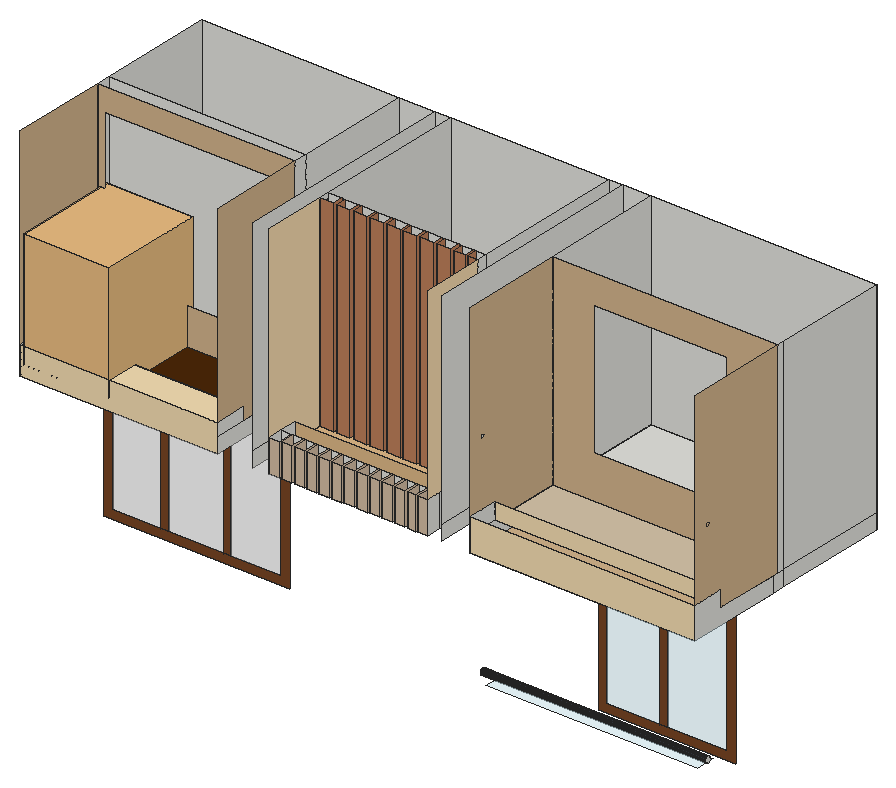
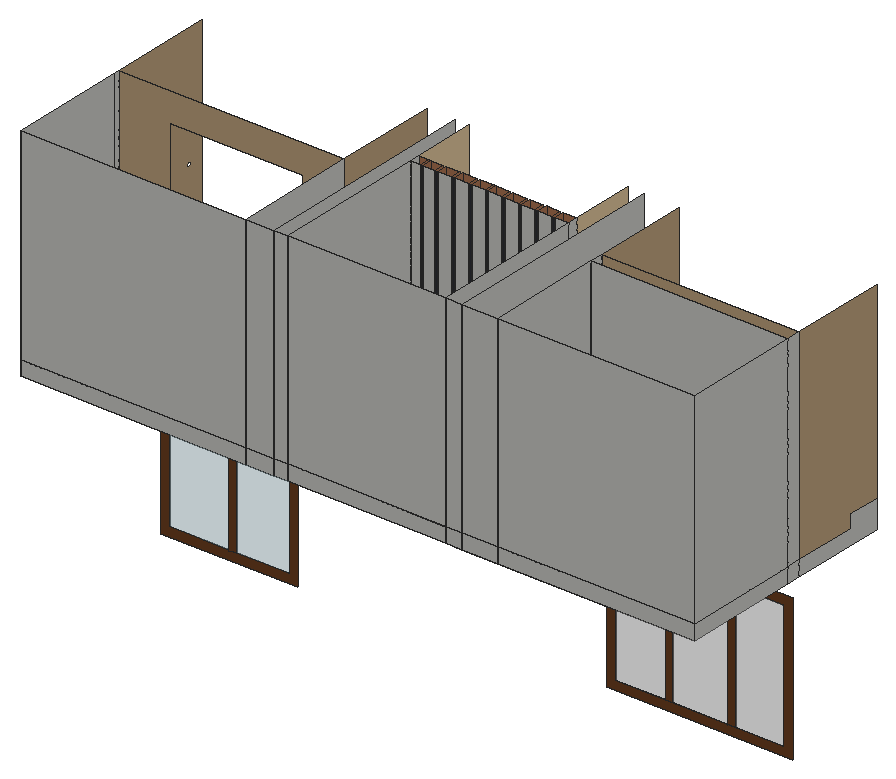
# SketchUp Ruby script. Lengths in inches.
U = 1.inch
M = Sketchup.active_model
def pt(a) = Geom::Point3d.new(a.map { |v| v * U })
def face(e, loops, mat)
  f = e.add_face(loops[0].map { |a| pt(a) })
  loops[1..].each { |l| e.add_face(l.map { |a| pt(a) }).erase! }
  f.material = f.back_material = mat if mat
  f
end
# faces: each face lists its corners as indices into pts; further lists are holes
def faces(e, pts, list, mat = nil) = list.each { |f| face(e, (f[0].is_a?(Array) ? f : [f]).map { |l| l.map { |i| pts[i] } }, mat) }
# xy, xz, yz: faces in a plane at the given z, y or x. An outline is a flat list of corners, or four numbers for a rectangle; further outlines are holes
def ring(l) = l.size == 4 ? [[l[0], l[1]], [l[2], l[1]], [l[2], l[3]], [l[0], l[3]]] : l.each_slice(2).to_a
def flat(e, list, mat, &to3) = list.each { |f| face(e, (f[0].is_a?(Array) ? f : [f]).map { |l| ring(l).map { |u, v| to3.(u, v) } }, mat) }
def xy(e, z, list, mat = nil) = flat(e, list, mat) { |x, y| [x, y, z] }
def xz(e, y, list, mat = nil) = flat(e, list, mat) { |x, z| [x, y, z] }
def yz(e, x, list, mat = nil) = flat(e, list, mat) { |y, z| [x, y, z] }
def lines(e, pts, list) = list.each { |a, b| e.add_line(pt(pts[a]), pt(pts[b])) }
# prism: a flat outline (further loops are holes) pulled along v
def prism(e, loops, v, mat = nil)
  f = face(e, loops, mat); d = Geom::Vector3d.new(v.map { |x| x * U })
  f.pushpull(f.normal.samedirection?(d) ? d.length : -d.length)
end
def box(e, o, s, mat = nil) = prism(e, [[o, [o[0] + s[0], o[1], o[2]], [o[0] + s[0], o[1] + s[1], o[2]], [o[0], o[1] + s[1], o[2]]]], [0, 0, s[2]], mat)
def at(x, y, z, deg = 0) = Geom::Transformation.translation(pt([x, y, z])) * Geom::Transformation.rotation(ORIGIN, Z_AXIS, deg.degrees)
def axes(o, x, y, z) = Geom::Transformation.new([*x, 0, *y, 0, *z, 0, *pt(o).to_a, 1])
def part(name) = M.definitions.add(name)
# library, detail: a bought-in or finely detailed component or shape, given as its bounding box
def library(name, o, s) = part(name).tap { |d| box(d.entities, o, s) }
def detail(e, o, s) = box(e.add_group.entities, o, s)
def put(e, d, t, mat = nil) = e.add_instance(d, t).tap { |i| i.material = mat if mat }
def group(e, t, mat = nil) = e.add_group.tap { |g| g.transformation = t; g.material = mat if mat }.entities
root = M.entities
M.materials.add("[0027_PeachPuff]").color = [255, 218, 185]
M.materials.add("[0034_Wheat]").color = [245, 222, 179]
M.materials.add("[0035_Tan]").color = [210, 180, 140]
M.materials.add("[0036_BurlyWood]1").color = [222, 184, 135]
M.materials.add("[Formica Beige]").color = [247, 219, 174]
M.materials.add("[Formica Laminate Dark]").color = [50, 53, 60]
M.materials.add("[Formica Laminate Light]").color = [213, 189, 164]
M.materials.add("[Leather Red Brown]").color = [76, 40, 8]
M.materials.add("[Tile Various Tan]").color = [214, 196, 169]
M.materials.add("[Translucent Glass Gray]").color = [191, 191, 191]
M.materials["[Translucent Glass Gray]"].alpha = 0.5
M.materials.add("[Translucent Glass Safety]").color = [204, 235, 244]
M.materials["[Translucent Glass Safety]"].alpha = 0.5
M.materials.add("[Wood Veneer 01]").color = [120, 70, 37]
M.materials.add("[Wood Veneer 02]").color = [190, 128, 91]
c1 = library("chau cay",[-24.34,-109.24,0],[56.46,62.58,79.69])
xy(root,3433.875,[[1418.67,332.12,2047.84,393.82]],"[Translucent Glass Safety]")
xy(root,3459.4375,[[2057.02,340.46,2059.25,340.76,2061.33,341.62,2063.12,342.99,2064.49,344.77,2065.35,346.85,2065.64,349.09,2065.35,351.32,2064.6,353.14,2049.4375,353.14,2048.6875,351.32,2048.39,349.09,2048.6875,346.85,2049.55,344.77,2050.92,342.99,2052.7,341.62,2054.79,340.76],[2049.4375,353.14,2064.6,353.14,2064.49,353.4,2063.12,355.1875,2061.33,356.56,2059.25,357.42,2057.02,357.71,2054.79,357.42,2052.7,356.56,2050.92,355.1875,2049.55,353.4]])
xy(root,3461.67,[[1409.52,340.46,1411.75,340.76,1413.83,341.62,1415.62,342.99,1416.99,344.77,1417.85,346.85,1418.14,349.09,1417.85,351.32,1417.22,352.84,1401.82,352.84,1401.1875,351.32,1400.89,349.09,1401.1875,346.85,1402.05,344.77,1403.42,342.99,1405.2,341.62,1407.29,340.76],[1401.82,352.84,1417.22,352.84,1416.99,353.4,1415.62,355.1875,1413.83,356.56,1411.75,357.42,1409.52,357.71,1407.29,357.42,1405.2,356.56,1403.42,355.1875,1402.05,353.4]])
xy(root,3798.8125,[[800.41,509.42,800.41,584.29,1272.8,584.29,1272.8,548.04,1258.16,548.04,1258.16,509.42,1201.66,509.42,1201.66,548.04,1191.29,548.04,1191.29,509.42,1134.78,509.42,1134.78,548.04,1124.41,548.04,1124.41,509.42,1067.91,509.42,1067.91,548.04,1057.54,548.04,1057.54,509.42,1001.03,509.42,1001.03,548.04,990.66,548.04,990.66,509.42,934.16,509.42,934.16,548.04,923.79,548.04,923.79,509.42,867.28,509.42,867.28,548.04,856.91,548.04,856.91,509.42],[800.41,509.42,856.91,548.04],[867.28,509.42,923.79,548.04],[934.16,509.42,990.66,548.04],[1001.03,509.42,1057.54,548.04],
  [1067.91,509.42,1124.41,548.04],[1134.78,509.42,1191.29,548.04],[1201.66,509.42,1258.16,548.04],[800.41,548.04,1272.8,584.29],[58.44,584.29,646.67,623.89],
  [646.67,584.29,752.97,623.89],[752.97,584.29,800.41,623.89],[800.41,584.29,1272.8,623.89],[1272.8,584.29,1313.62,623.89],[1272.8,584.29,1313.62,623.89],
  [1313.62,584.29,1398.32,623.89],[58.44,623.89,646.67,971.67],[646.67,623.89,752.97,971.67],[752.97,623.89,800.41,971.67],[800.41,623.89,1272.8,971.67],
  [1272.8,623.89,1313.62,971.67],[1313.62,623.89,1398.32,971.67],[1398.32,623.89,2069.85,971.67]])
xy(root,3798.8125,[[800.41,338.63,800.41,509.42,856.91,509.42,856.91,548.04,867.28,548.04,867.28,509.42,923.79,509.42,923.79,548.04,934.16,548.04,934.16,509.42,990.66,509.42,990.66,548.04,1001.03,548.04,1001.03,509.42,1057.54,509.42,1057.54,548.04,1067.91,548.04,1067.91,509.42,1124.41,509.42,1124.41,548.04,1134.78,548.04,1134.78,509.42,1191.29,509.42,1191.29,548.04,1201.66,548.04,1201.66,509.42,1258.16,509.42,1258.16,548.04,1272.8,548.04,1272.8,338.63]],"[0027_PeachPuff]")
xy(root,3798.8125,[[58.44,295.82,646.67,584.29],[1398.32,295.82,2069.85,584.29],[1398.32,584.29,2069.85,623.89]],"[0035_Tan]")
xy(root,3798.8125,[[800.41,295.82,831.22,338.63],[837.47,295.82,868.28,338.63],[875.6,295.82,906.41,338.63],[912.41,295.82,943.22,338.63],[949.16,295.82,979.97,338.63],
  [986.78,295.82,1017.6,338.63],[1024.35,295.82,1055.16,338.63],[1062.53,295.82,1093.35,338.63],[1100.28,295.82,1131.1,338.63],[1137.66,295.82,1168.47,338.63],
  [1175.22,295.82,1206.03,338.63],[1212.97,295.82,1238.19,338.63],[1243.78,295.82,1272.8,338.63]],"[Formica Laminate Light]")
xy(root,3844,[[800.41,483.92,841.6875,514.17],[850.41,483.92,891.6875,514.17],[900.97,483.92,942.25,514.17],[949.72,483.92,991,514.17],[1000.6,483.92,1041.875,514.17],
  [1049.35,483.92,1090.625,514.17],[1099.6,483.92,1140.875,514.17],[1149.66,483.92,1190.9375,514.17],[1200.46,483.92,1235.22,514.17],[1241.74,483.92,1272.8,514.17],
  [800.41,514.17,1272.8,971.67],[58.44,584.29,646.67,623.89],[1398.32,604.09,2069.85,971.67],[58.44,623.89,646.67,971.67]])
xy(root,3844,[[800.41,390.27,1272.8,390.27,1272.8,483.92,1241.74,483.92,1241.74,514.17,1235.22,514.17,1235.22,483.92,1200.46,483.92,1200.46,514.17,1190.9375,514.17,1190.9375,483.92,1149.66,483.92,1149.66,514.17,1140.875,514.17,1140.875,483.92,1099.6,483.92,1099.6,514.17,1090.625,514.17,1090.625,483.92,1049.35,483.92,1049.35,514.17,1041.875,514.17,1041.875,483.92,1000.6,483.92,1000.6,514.17,991,514.17,991,483.92,949.72,483.92,949.72,514.17,942.25,514.17,942.25,483.92,900.97,483.92,900.97,514.17,891.6875,514.17,891.6875,483.92,850.41,483.92,850.41,514.17,841.6875,514.17,841.6875,483.92,800.41,483.92]],"[0036_BurlyWood]1")
xy(root,3844,[[58.44,390.27,646.67,584.29]],"[Leather Red Brown]")
xy(root,3844,[[1398.32,390.27,2069.85,604.09]],"[Tile Various Tan]")
xy(root,3881.75,[[58.44,295.82,646.67,390.27]],"[0034_Wheat]")
xz(root,295.82,[[58.44,3798.8125,646.67,3881.75],[1398.32,3798.8125,2069.85,3893.0625]],"[0034_Wheat]")
xz(root,295.82,[[800.41,3798.8125,831.22,3896.1875],[837.47,3798.8125,868.28,3896.1875],[875.6,3798.8125,906.41,3896.1875],[912.41,3798.8125,943.22,3896.1875],[949.16,3798.8125,979.97,3896.1875],
  [986.78,3798.8125,1017.6,3896.1875],[1024.35,3798.8125,1055.16,3896.1875],[1062.53,3798.8125,1093.35,3896.1875],[1100.28,3798.8125,1131.1,3896.1875],[1137.66,3798.8125,1168.47,3896.1875],
  [1175.22,3798.8125,1206.03,3896.1875],[1212.97,3798.8125,1238.19,3896.1875],[1243.78,3798.8125,1272.8,3896.1875]],"[Formica Laminate Light]")
xz(root,338.63,[[800.41,3798.8125,831.22,3896.1875],[837.47,3798.8125,868.28,3896.1875],[875.6,3798.8125,906.41,3896.1875],[912.41,3798.8125,943.22,3896.1875],[949.16,3798.8125,979.97,3896.1875],
  [986.78,3798.8125,1017.6,3896.1875],[1024.35,3798.8125,1055.16,3896.1875],[1062.53,3798.8125,1093.35,3896.1875],[1100.28,3798.8125,1131.1,3896.1875],[1137.66,3798.8125,1168.47,3896.1875],
  [1175.22,3798.8125,1206.03,3896.1875],[1212.97,3798.8125,1238.19,3896.1875],[1243.78,3798.8125,1272.8,3896.1875]])
xz(root,338.63,[[831.22,3798.8125,837.47,3896.1875],[868.28,3798.8125,875.6,3896.1875],[906.41,3798.8125,912.41,3896.1875],[943.22,3798.8125,949.16,3896.1875],[979.97,3798.8125,986.78,3896.1875],
  [1017.6,3798.8125,1024.35,3896.1875],[1055.16,3798.8125,1062.53,3896.1875],[1093.35,3798.8125,1100.28,3896.1875],[1131.1,3798.8125,1137.66,3896.1875],[1168.47,3798.8125,1175.22,3896.1875],
  [1206.03,3798.8125,1212.97,3896.1875],[1238.19,3798.8125,1243.78,3896.1875]],"[Formica Laminate Dark]")
xz(root,390.27,[[58.44,3844,646.67,3881.75]])
xz(root,390.27,[[1398.32,3844,2069.85,3893.0625]],"[0034_Wheat]")
xz(root,390.27,[[800.41,3844,1272.8,3896.1875]],"[0036_BurlyWood]1")
xz(root,483.92,[[800.41,3844,841.6875,4453.25],[850.41,3844,891.6875,4453.25],[900.97,3844,942.25,4453.25],[949.72,3844,991,4453.25],[1000.6,3844,1041.875,4453.25],
  [1049.35,3844,1090.625,4453.25],[1099.6,3844,1140.875,4453.25],[1149.66,3844,1190.9375,4453.25],[1200.46,3844,1235.22,4453.25],[1241.74,3844,1272.8,4453.25]],"[Wood Veneer 02]")
xz(root,514.17,[[800.41,3844,841.6875,4453.25],[850.41,3844,891.6875,4453.25],[900.97,3844,942.25,4453.25],[949.72,3844,991,4453.25],[1000.6,3844,1041.875,4453.25],
  [1049.35,3844,1090.625,4453.25],[1099.6,3844,1140.875,4453.25],[1149.66,3844,1190.9375,4453.25],[1200.46,3844,1235.22,4453.25],[1241.74,3844,1272.8,4453.25]])
xz(root,514.17,[[841.6875,3844,850.41,4453.25],[891.6875,3844,900.97,4453.25],[942.25,3844,949.72,4453.25],[991,3844,1000.6,4453.25],[1041.875,3844,1049.35,4453.25],
  [1090.625,3844,1099.6,4453.25],[1140.875,3844,1149.66,4453.25],[1190.9375,3844,1200.46,4453.25],[1235.22,3844,1241.74,4453.25]],"[Formica Laminate Dark]")
xz(root,584.29,[[[58.44,3844,646.67,4453.25],[80.45,3953.99,630.58,4386.93]]],"[0035_Tan]")
xz(root,584.29,[[102.12,3330.58,247.0625,3710.59],[269.68,3330.58,433.0625,3710.59],[455.68,3330.58,604.93,3710.59]],"[Translucent Glass Gray]")
xz(root,584.29,[[[76.9,3305.37,630.15,3735.8],[102.12,3330.58,604.93,3710.59]],[247.0625,3330.58,269.68,3710.59],[433.0625,3330.58,455.68,3710.59]],"[Wood Veneer 01]")
xz(root,604.09,[[[1398.32,3844,2069.85,4453.25],[1523.05,3973.96,1917.8,4368.71]]],"[0035_Tan]")
xz(root,623.89,[[58.44,3844,646.67,4453.25]])
xz(root,623.89,[[1546.07,3301.52,1703.52,3696.56],[1725.625,3301.52,1903.36,3696.56]],"[Translucent Glass Safety]")
xz(root,623.89,[[[1520.9,3276.35,1928.53,3721.73],[1546.07,3301.52,1903.36,3696.56]],[1703.52,3301.52,1725.625,3696.56]],"[Wood Veneer 01]")
xz(root,971.67,[[58.44,3798.8125,646.67,3844],[646.67,3798.8125,752.97,3844],[752.97,3798.8125,800.41,3844],[800.41,3798.8125,1272.8,3844],[1272.8,3798.8125,1313.62,3844],
  [1313.62,3798.8125,1398.32,3844],[1398.32,3798.8125,2069.85,3844],[58.44,3844,646.67,4453.25],[646.67,3844,752.97,4453.25],[752.97,3844,800.41,4453.25],
  [800.41,3844,1272.8,4453.25],[1272.8,3844,1313.62,4453.25],[1313.62,3844,1398.32,4453.25],[1398.32,3844,2069.85,4453.25]])
yz(root,58.44,[[295.82,3798.8125,295.82,3881.75,390.27,3881.75,390.27,3844,584.29,3844,584.29,3798.8125],[584.29,3798.8125,623.89,3844],[623.89,3798.8125,971.67,3844],[584.29,3844,623.89,4453.25],[623.89,3844,971.67,4453.25]])
yz(root,58.44,[[390.27,3844,584.29,3844,584.29,4453.25,295.82,4453.25,295.82,3881.75,390.27,3881.75]],"[0035_Tan]")
yz(root,646.67,[[295.82,3798.8125,971.67,3844],[295.82,3844,390.27,3881.75],[584.29,3844,623.89,4453.25],[623.89,3844,971.67,4453.25]])
yz(root,646.67,[[390.27,3844,390.27,3881.75,295.82,3881.75,295.82,4453.25,584.29,4453.25,584.29,3844]],"[0035_Tan]")
yz(root,752.97,[[295.82,3798.8125,971.67,3844],[295.82,3844,971.67,4453.25]])
yz(root,800.41,[[295.82,3798.8125,338.63,3896.1875],[338.63,3798.8125,971.67,3798.8125,971.67,3844,390.27,3844,390.27,3896.1875,338.63,3896.1875],[483.92,3844,514.17,4453.25],[514.17,3844,971.67,4453.25]])
yz(root,800.41,[[390.27,3844,483.92,3844,483.92,4453.25,295.82,4453.25,295.82,3896.1875,390.27,3896.1875]],"[Formica Beige]")
yz(root,831.22,[[295.82,3798.8125,338.63,3896.1875]],"[Formica Laminate Light]")
yz(root,837.47,[[295.82,3798.8125,338.63,3896.1875]],"[Formica Laminate Light]")
yz(root,841.6875,[[483.92,3844,514.17,4453.25]],"[Wood Veneer 02]")
yz(root,850.41,[[483.92,3844,514.17,4453.25]],"[Wood Veneer 02]")
yz(root,868.28,[[295.82,3798.8125,338.63,3896.1875]],"[Formica Laminate Light]")
yz(root,875.6,[[295.82,3798.8125,338.63,3896.1875]],"[Formica Laminate Light]")
yz(root,891.6875,[[483.92,3844,514.17,4453.25]],"[Wood Veneer 02]")
yz(root,900.97,[[483.92,3844,514.17,4453.25]],"[Wood Veneer 02]")
yz(root,906.41,[[295.82,3798.8125,338.63,3896.1875]],"[Formica Laminate Light]")
yz(root,912.41,[[295.82,3798.8125,338.63,3896.1875]],"[Formica Laminate Light]")
yz(root,942.25,[[483.92,3844,514.17,4453.25]],"[Wood Veneer 02]")
yz(root,943.22,[[295.82,3798.8125,338.63,3896.1875]],"[Formica Laminate Light]")
yz(root,949.16,[[295.82,3798.8125,338.63,3896.1875]],"[Formica Laminate Light]")
yz(root,949.72,[[483.92,3844,514.17,4453.25]],"[Wood Veneer 02]")
yz(root,979.97,[[295.82,3798.8125,338.63,3896.1875]],"[Formica Laminate Light]")
yz(root,986.78,[[295.82,3798.8125,338.63,3896.1875]],"[Formica Laminate Light]")
yz(root,991,[[483.92,3844,514.17,4453.25]],"[Wood Veneer 02]")
yz(root,1000.6,[[483.92,3844,514.17,4453.25]],"[Wood Veneer 02]")
yz(root,1017.6,[[295.82,3798.8125,338.63,3896.1875]],"[Formica Laminate Light]")
yz(root,1024.35,[[295.82,3798.8125,338.63,3896.1875]],"[Formica Laminate Light]")
yz(root,1041.875,[[483.92,3844,514.17,4453.25]],"[Wood Veneer 02]")
yz(root,1049.35,[[483.92,3844,514.17,4453.25]],"[Wood Veneer 02]")
yz(root,1055.16,[[295.82,3798.8125,338.63,3896.1875]],"[Formica Laminate Light]")
yz(root,1062.53,[[295.82,3798.8125,338.63,3896.1875]],"[Formica Laminate Light]")
yz(root,1090.625,[[483.92,3844,514.17,4453.25]],"[Wood Veneer 02]")
yz(root,1093.35,[[295.82,3798.8125,338.63,3896.1875]],"[Formica Laminate Light]")
yz(root,1099.6,[[483.92,3844,514.17,4453.25]],"[Wood Veneer 02]")
yz(root,1100.28,[[295.82,3798.8125,338.63,3896.1875]],"[Formica Laminate Light]")
yz(root,1131.1,[[295.82,3798.8125,338.63,3896.1875]],"[Formica Laminate Light]")
yz(root,1137.66,[[295.82,3798.8125,338.63,3896.1875]],"[Formica Laminate Light]")
yz(root,1140.875,[[483.92,3844,514.17,4453.25]],"[Wood Veneer 02]")
yz(root,1149.66,[[483.92,3844,514.17,4453.25]],"[Wood Veneer 02]")
yz(root,1168.47,[[295.82,3798.8125,338.63,3896.1875]],"[Formica Laminate Light]")
yz(root,1175.22,[[295.82,3798.8125,338.63,3896.1875]],"[Formica Laminate Light]")
yz(root,1190.9375,[[483.92,3844,514.17,4453.25]],"[Wood Veneer 02]")
yz(root,1200.46,[[483.92,3844,514.17,4453.25]],"[Wood Veneer 02]")
yz(root,1206.03,[[295.82,3798.8125,338.63,3896.1875]],"[Formica Laminate Light]")
yz(root,1212.97,[[295.82,3798.8125,338.63,3896.1875]],"[Formica Laminate Light]")
yz(root,1235.22,[[483.92,3844,514.17,4453.25]],"[Wood Veneer 02]")
yz(root,1238.19,[[295.82,3798.8125,338.63,3896.1875]],"[Formica Laminate Light]")
yz(root,1241.74,[[483.92,3844,514.17,4453.25]],"[Wood Veneer 02]")
yz(root,1243.78,[[295.82,3798.8125,338.63,3896.1875]],"[Formica Laminate Light]")
yz(root,1272.8,[[295.82,3798.8125,338.63,3896.1875],[338.63,3798.8125,338.63,3896.1875,390.27,3896.1875,390.27,3844,971.67,3844,971.67,3798.8125],[483.92,3844,514.17,4453.25],[514.17,3844,971.67,4453.25]])
yz(root,1272.8,[[390.27,3844,390.27,3896.1875,295.82,3896.1875,295.82,4453.25,483.92,4453.25,483.92,3844]],"[Formica Beige]")
yz(root,1313.62,[[295.82,3798.8125,971.67,3844],[295.82,3844,971.67,4453.25]])
yz(root,1398.32,[[295.82,3798.8125,971.67,3844],[295.82,3844,390.27,3893.0625],[604.09,3844,971.67,4453.25]])
yz(root,1398.32,[[[390.27,3844,604.09,3844,604.09,4453.25,295.82,4453.25,295.82,3893.0625,390.27,3893.0625],[343.39,4082.13,341.61,4082.37,339.95,4083.05,338.53,4084.15,337.4375,4085.57,336.75,4087.23,336.52,4089.01,336.75,4090.79,337.4375,4092.45,338.53,4093.87,339.95,4094.96,341.61,4095.65,343.39,4095.88,345.17,4095.65,346.83,4094.96,348.25,4093.87,349.34,4092.45,350.03,4090.79,350.27,4089.01,350.03,4087.23,349.34,4085.57,348.25,4084.15,346.83,4083.05,345.17,4082.37]]],"[0035_Tan]")
yz(root,2069.85,[[344.51,3450.8125,346.74,3451.11,348.82,3451.97,350.61,3453.34,351.98,3455.125,352.84,3457.21,353.14,3459.4375,352.84,3461.67,351.98,3463.75,350.61,3465.54,348.82,3466.91,346.74,3467.77,344.51,3468.0625,342.28,3467.77,340.2,3466.91,338.41,3465.54,337.04,3463.75,336.18,3461.67,335.89,3459.4375,336.18,3457.21,337.04,3455.125,338.41,3453.34,340.2,3451.97,342.28,3451.11],[295.82,3798.8125,584.29,3798.8125,584.29,3844,390.27,3844,390.27,3893.0625,295.82,3893.0625],[584.29,3798.8125,623.89,3844],[623.89,3798.8125,971.67,3844],[604.09,3844,623.89,4453.25],
  [623.89,3844,971.67,4453.25]])
yz(root,2069.85,[[[390.27,3844,390.27,3893.0625,295.82,3893.0625,295.82,4453.25,604.09,4453.25,604.09,3844],[343.39,4082.13,345.17,4082.37,346.83,4083.05,348.25,4084.15,349.34,4085.57,350.03,4087.23,350.27,4089.01,350.03,4090.79,349.34,4092.45,348.25,4093.87,346.83,4094.96,345.17,4095.65,343.39,4095.88,341.61,4095.65,339.95,4094.96,338.53,4093.87,337.4375,4092.45,336.75,4090.79,336.52,4089.01,336.75,4087.23,337.4375,4085.57,338.53,4084.15,339.95,4083.05,341.61,4082.37]]],"[0035_Tan]")
p = [[2069.85,344.51,3450.8125],[2069.85,342.28,3451.11],[1398.32,342.28,3451.11],[1398.32,344.51,3450.8125],[2069.85,346.74,3451.11],[1398.32,346.74,3451.11],
  [2069.85,340.2,3451.97],[1398.32,340.2,3451.97],[2069.85,348.82,3451.97],[1398.32,348.82,3451.97],[2069.85,338.41,3453.34],[1398.32,338.41,3453.34],
  [2069.85,350.61,3453.34],[1398.32,350.61,3453.34],[2069.85,337.04,3455.125],[1398.32,337.04,3455.125],[2069.85,351.98,3455.125],[1398.32,351.98,3455.125],
  [2069.85,336.18,3457.21],[1398.32,336.18,3457.21],[2069.85,352.84,3457.21],[1398.32,352.84,3457.21],[2069.85,335.89,3459.4375],[1398.32,335.89,3459.4375],
  [2069.85,353.14,3459.4375],[1398.32,353.14,3459.4375],[2049.4375,353.14,3459.4375],[2064.6,353.14,3459.4375],[2069.85,336.18,3461.67],[1398.32,336.18,3461.67],
  [2069.85,352.84,3461.67],[1398.32,352.84,3461.67],[1401.82,352.84,3461.67],[1417.22,352.84,3461.67],[2069.85,337.04,3463.75],[1398.32,337.04,3463.75],
  [2069.85,351.98,3463.75],[1398.32,351.98,3463.75],[2069.85,338.41,3465.54],[1398.32,338.41,3465.54],[2069.85,350.61,3465.54],[1398.32,350.61,3465.54],
  [2069.85,340.2,3466.91],[1398.32,340.2,3466.91],[2069.85,348.82,3466.91],[1398.32,348.82,3466.91],[2069.85,342.28,3467.77],[1398.32,342.28,3467.77],
  [2069.85,346.74,3467.77],[1398.32,346.74,3467.77],[2069.85,344.51,3468.0625],[1398.32,344.51,3468.0625]]
faces(root,p,[[0,1,2,3],[4,0,3,5],[1,6,7,2],[8,4,5,9],[6,10,11,7],[12,8,9,13],[10,14,15,11],[16,12,13,17],
  [14,18,19,15],[20,16,17,21],[18,22,23,19],[24,20,21,25,26,27],[22,28,29,23],[30,24,27,26,25,31,32,33],[28,34,35,29],[36,30,33,32,31,37],
  [34,38,39,35],[40,36,37,41],[38,42,43,39],[44,40,41,45],[42,46,47,43],[48,44,45,49],[46,50,51,47],[50,48,49,51]],"[Formica Laminate Dark]")
put(root,c1,axes([178.4,64.16,3833.82],[4.5,0,0],[0,-4.9651,0],[0,0,4.37432]))
